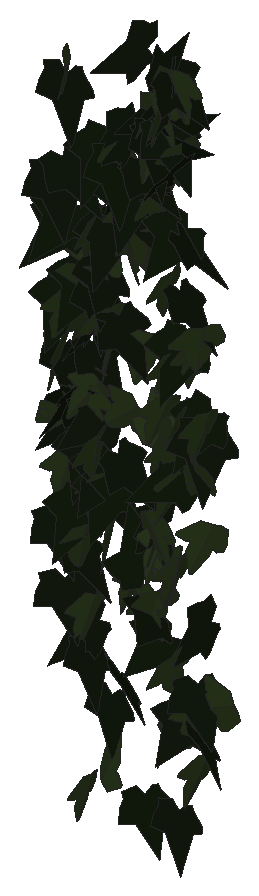
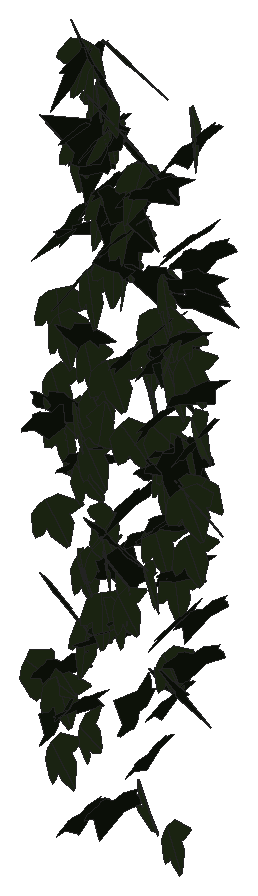
# SketchUp Ruby script. Lengths in inches.
U = 1.inch
M = Sketchup.active_model
def pt(a) = Geom::Point3d.new(a.map { |v| v * U })
def face(e, loops, mat)
  f = e.add_face(loops[0].map { |a| pt(a) })
  loops[1..].each { |l| e.add_face(l.map { |a| pt(a) }).erase! }
  f.material = f.back_material = mat if mat
  f
end
# faces: each face lists its corners as indices into pts; further lists are holes
def faces(e, pts, list, mat = nil) = list.each { |f| face(e, (f[0].is_a?(Array) ? f : [f]).map { |l| l.map { |i| pts[i] } }, mat) }
# xy, xz, yz: faces in a plane at the given z, y or x. An outline is a flat list of corners, or four numbers for a rectangle; further outlines are holes
def ring(l) = l.size == 4 ? [[l[0], l[1]], [l[2], l[1]], [l[2], l[3]], [l[0], l[3]]] : l.each_slice(2).to_a
def flat(e, list, mat, &to3) = list.each { |f| face(e, (f[0].is_a?(Array) ? f : [f]).map { |l| ring(l).map { |u, v| to3.(u, v) } }, mat) }
def xy(e, z, list, mat = nil) = flat(e, list, mat) { |x, y| [x, y, z] }
def xz(e, y, list, mat = nil) = flat(e, list, mat) { |x, z| [x, y, z] }
def yz(e, x, list, mat = nil) = flat(e, list, mat) { |y, z| [x, y, z] }
def lines(e, pts, list) = list.each { |a, b| e.add_line(pt(pts[a]), pt(pts[b])) }
# prism: a flat outline (further loops are holes) pulled along v
def prism(e, loops, v, mat = nil)
  f = face(e, loops, mat); d = Geom::Vector3d.new(v.map { |x| x * U })
  f.pushpull(f.normal.samedirection?(d) ? d.length : -d.length)
end
def box(e, o, s, mat = nil) = prism(e, [[o, [o[0] + s[0], o[1], o[2]], [o[0] + s[0], o[1] + s[1], o[2]], [o[0], o[1] + s[1], o[2]]]], [0, 0, s[2]], mat)
def at(x, y, z, deg = 0) = Geom::Transformation.translation(pt([x, y, z])) * Geom::Transformation.rotation(ORIGIN, Z_AXIS, deg.degrees)
def axes(o, x, y, z) = Geom::Transformation.new([*x, 0, *y, 0, *z, 0, *pt(o).to_a, 1])
def part(name) = M.definitions.add(name)
# library, detail: a bought-in or finely detailed component or shape, given as its bounding box
def library(name, o, s) = part(name).tap { |d| box(d.entities, o, s) }
def detail(e, o, s) = box(e.add_group.entities, o, s)
def put(e, d, t, mat = nil) = e.add_instance(d, t).tap { |i| i.material = mat if mat }
def group(e, t, mat = nil) = e.add_group.tap { |g| g.transformation = t; g.material = mat if mat }.entities
root = M.entities
M.materials.add("efeu1").color = [18, 25, 13]
M.materials.add("efeu2").color = [43, 57, 29]
c1 = part("ivyleaf_10")
p = [[0,0.5,-0.03],[-0.0625,2.02,-0.43],[-0.19,2.01,-0.46],[-0.54,1.05,-0.29],[-0.52,0.625,-0.18],[-0.83,0.76,-0.28],
  [-1.16,0.64,-0.33],[-1.15,0.33,-0.24],[-0.77,-0.39,0.02],[-0.3,-0.51,0.16],[0.04,-0.48,0.23],[-0.02,2.01,-0.4375],
  [-0.06,2.01,-0.43],[0.04,-0.49,0.23],[0.67,-0.49,0.14],[1.38,0.36,-0.2],[1.375,0.51,-0.24],[0.81,0.65,-0.19],
  [0.62,0.59,-0.15],[0.6,1.09,-0.28],[0.5,1.23,-0.31]]
faces(c1.entities,p,[[0,1,2,3,4,5,6,7,8,9,10],[11,12,0,13,14,15,16,17,18,19,20]],"efeu2")
c2 = part("ivyleaf_9")
p = [[1.54,2.16,1.25],[1.36,2.04,1.19],[-0.21,0.99,0.68],[-0.71,1.11,0.82],[-0.85,0.86,0.67],[-0.8,0.17,0.21],
  [-0.9,-0.01,0.1],[-0.67,-0.16,-0.02],[-0.08,-0.08,-0.05],[-0.03,-0.6,-0.4],[0.65,-0.88,-0.66],[0.83,-0.6,-0.49],
  [1.29,-0.42,-0.43],[1.8125,-0.07,-0.26],[1.21,0.44,0.15]]
faces(c2.entities,p,[[0,1,2,3,4,5,6,7,8,9,10,11,12,13,14]],"efeu1")
put(root,c1,axes([526.16,131.21,239.89],[0.45745,-0.87487,-0.09808],[0.01557,0.11855,-0.98488],[0.88021,0.45257,0.06839]))
put(root,c1,axes([522.93,131.16,223.58],[0.0269,-0.92071,-0.14302],[0.00472,0.14321,-0.92106],[0.93174,0.02586,0.00879]))
put(root,c2,axes([521.15,131.58,239.56],[0.07665,-0.98925,-0.02502],[-0.01925,0.0236,-0.99206],[0.98938,0.0771,-0.01737]))
put(root,c2,axes([524.41,131.73,235.49],[-0.2445,-0.93887,0.09298],[-0.00632,-0.09442,-0.97003],[0.94344,-0.24395,0.0176]))
put(root,c1,axes([526.94,131.03,214.93],[-0.1751,-0.89884,-0.3085],[0.08375,0.29787,-0.91543],[0.94661,-0.19262,0.02393]))
put(root,c2,axes([525.29,131.9,216.17],[-0.26022,-0.64301,0.58185],[0.22645,-0.63679,-0.60245],[0.8371,-0.02762,0.34385]))
put(root,c1,axes([526.52,130.88,225.14],[0.21684,-0.73874,-0.54662],[0.13314,0.58096,-0.73233],[0.90929,0.09111,0.23758]))
put(root,c2,axes([523.6875,131.62,236.61],[-0.02137,-0.98061,-0.09477],[0.00149,0.09476,-0.98084],[0.98517,-0.02142,-0.00057]))
put(root,c2,axes([525.63,131.67,238.39],[0.16649,-0.97049,0.06718],[-0.00025,-0.0682,-0.98459],[0.97281,0.16608,-0.01175]))
put(root,c2,axes([522.27,131.58,213.65],[0.14457,-0.87641,-0.02007],[-0.00231,0.01996,-0.88825],[0.87664,0.14458,0.00097]))
put(root,c2,axes([523.02,131.86,236.97],[-0.50649,-0.83413,0.08884],[0.03508,-0.12475,-0.97129],[0.83811,-0.49886,0.09434]))
put(root,c2,axes([521.68,131.92,219.92],[-0.42513,-0.8034,0.19731],[-0.05961,-0.19151,-0.90823],[0.82512,-0.42778,0.03605]))
put(root,c2,axes([526.93,130.72,237.33],[0.00765,0.95187,0.24437],[-0.01575,0.24446,-0.95175],[-0.98261,0.00349,0.01716]))
put(root,c2,axes([525.27,131.4,242.33],[-0.87542,0.45236,0.16553],[-0.20762,-0.04451,-0.97638],[-0.43466,-0.88982,0.133]))
put(root,c1,axes([521.4,131.19,240.36],[0.5028,-0.78984,-0.35606],[-0.0926,0.36033,-0.93007],[0.86143,0.49975,0.10784]))
put(root,c2,axes([524.31,131.49,238.12],[-0.94168,0.27966,-0.00731],[0.0064,-0.00414,-0.98232],[-0.27968,-0.9417,0.00214]))
put(root,c1,axes([528.17,131.58,226.2],[-0.00795,-0.92129,0.17894],[0.0119,-0.17903,-0.92123],[0.93844,-0.00554,0.01319]))
put(root,c2,axes([525.91,132.05,215.29],[-0.59192,-0.5599,0.38395],[-0.0699,-0.45642,-0.77335],[0.67529,-0.53802,0.25649]))
put(root,c1,axes([522.13,131.42,219.07],[-0.22865,-0.88154,-0.0035],[0.00118,0.00331,-0.91071],[0.88154,-0.22865,0.00032]))
put(root,c2,axes([526.93,132.04,223.02],[-0.63851,-0.36043,0.60223],[-0.40913,-0.47038,-0.71529],[0.57026,-0.74103,0.16112]))
put(root,c1,axes([526.91,131.29,241.55],[-0.98612,0.08208,-0.12222],[0.1162,-0.07435,-0.98746],[-0.0904,-0.99088,0.06397]))
put(root,c2,axes([521.21,131.92,233.41],[-0.77924,-0.54246,0.1085],[-0.077,-0.07924,-0.94923],[0.54782,-0.78275,0.0209]))
put(root,c1,axes([525.39,131.63,238.45],[0.05897,0.89388,-0.41727],[-0.03025,-0.41618,-0.89582],[-0.98601,0.06622,0.00253]))
put(root,c2,axes([522.79,132.1,224.45],[-0.54463,-0.55878,0.4979],[-0.30959,-0.39242,-0.77905],[0.68139,-0.62492,0.044]))
put(root,c1,axes([522.49,131.91,225.86],[-0.28668,-0.62588,0.62813],[-0.19889,-0.59793,-0.68657],[0.86413,-0.34526,0.05036]))
put(root,c1,axes([526.04,131.75,226.17],[-0.13417,-0.8722,0.31137],[-0.05156,-0.3071,-0.88245],[0.92468,-0.14368,-0.00403]))
put(root,c1,axes([526.51,131.91,222.6875],[0.07964,-0.78186,0.49958],[0.05181,-0.49688,-0.78591],[0.92639,0.095,0.00101]))
put(root,c1,axes([521.16,131.79,229.31],[-0.12945,-0.90458,0.32863],[0.0044,-0.33215,-0.91251],[0.96241,-0.12015,0.04838]))
put(root,c1,axes([523.3,131.48,229.36],[-0.30349,-0.88514,-0.09861],[0.03706,0.09153,-0.93571],[0.88984,-0.3057,0.00534]))
put(root,c2,axes([526.84,132.17,211.86],[-0.40832,-0.71301,0.34579],[-0.03265,-0.37353,-0.80876],[0.79176,-0.38311,0.14497]))
put(root,c2,axes([520.53,131.76,234.875],[-0.15825,-0.9116,-0.31859],[0.08073,0.30922,-0.92489],[0.96229,-0.17585,0.0252]))
put(root,c2,axes([522.81,131.59,229.21],[-0.72667,0.60822,-0.28042],[0.18796,-0.21195,-0.94677],[-0.64284,-0.74951,0.04017]))
put(root,c1,axes([528.01,131.35,224.09],[-0.82191,0.08539,0.49093],[-0.48818,0.05186,-0.82633],[-0.0999,-0.95595,-0.00098]))
put(root,c2,axes([520.98,131.98,232.76],[-0.89275,-0.32041,0.09017],[-0.06278,-0.09139,-0.94631],[0.32688,-0.89263,0.06452]))
put(root,c1,axes([525.48,131.58,220.68],[-0.74831,0.31004,-0.44507],[0.37399,-0.25436,-0.80599],[-0.39287,-0.83268,0.08049]))
put(root,c2,axes([525.11,131.65,207.88],[0.00386,-0.78759,-0.37309],[-0.02363,0.37286,-0.78735],[0.87117,0.0136,-0.0197]))
put(root,c2,axes([523.03,132.11,221.29],[-0.38986,-0.8427,0.09054],[-0.00558,-0.09711,-0.92783],[0.84753,-0.38828,0.03554]))
put(root,c2,axes([523.59,131.98,212.78],[0.41557,-0.67224,0.50939],[0.29811,-0.41414,-0.78975],[0.789,0.51055,0.03009]))
put(root,c2,axes([521.77,132.22,230.41],[-0.51524,-0.78089,0.17721],[-0.02749,-0.19336,-0.93195],[0.80027,-0.5094,0.08209]))
put(root,c2,axes([521.85,131.46,225.18],[0.47545,0.57943,-0.60516],[-0.3701,-0.47899,-0.7494],[-0.75165,0.60236,-0.01379]))
put(root,c1,axes([522.04,131.8,207.45],[0.13598,-0.85125,0.13331],[0.04162,-0.12832,-0.8618],[0.86062,0.14071,0.02061]))
put(root,c1,axes([524.52,131.97,218.43],[0.015,-0.36595,-0.87914],[0.7619,-0.52283,0.23064],[-0.57124,-0.70694,0.28452]))
put(root,c1,axes([522.04,132,215.5],[-0.09112,-0.80566,0.38234],[0.12785,-0.39217,-0.79589],[0.88257,-0.02637,0.15477]))
put(root,c2,axes([520.88,131.81,216.23],[-0.11344,-0.81154,-0.36458],[0.13083,0.34832,-0.81605],[0.88,-0.1564,0.07433]))
put(root,c1,axes([522.06,131.59,225.28],[-0.88673,-0.05479,-0.25274],[0.25696,-0.08491,-0.88314],[0.02915,-0.91813,0.09676]))
put(root,c2,axes([526,131.62,239.68],[-0.8352,0.49732,0.17445],[-0.17095,0.05358,-0.9712],[-0.49853,-0.85154,0.04077]))
put(root,c1,axes([525.6,131.62,239.86],[-0.88626,0.22484,-0.37665],[0.3452,-0.16642,-0.9116],[-0.27066,-0.94848,0.07067]))
put(root,c2,axes([526.73,131.37,241.62],[0.35927,-0.60975,-0.70099],[-0.28636,0.64231,-0.70547],[0.88384,0.45596,0.05637]))
put(root,c2,axes([526.57,132.33,234.09],[-0.66559,-0.65359,0.21848],[0.02765,-0.32882,-0.89947],[0.68859,-0.61857,0.2473]))
put(root,c2,axes([528.21,131.83,216.87],[-0.94,0.24426,-0.14113],[0.13769,-0.03125,-0.9712],[-0.24621,-0.95002,-0.00434]))
put(root,c1,axes([527.9375,131.73,230],[-0.45804,-0.84692,0.04673],[-0.00526,-0.05027,-0.96265],[0.84819,-0.45767,0.01927]))
put(root,c2,axes([526.875,132.06,229.15],[-0.76516,-0.54241,-0.20354],[0.15941,0.12705,-0.93784],[0.55697,-0.78151,-0.0112]))
put(root,c2,axes([525.85,131.5625,240.76],[-0.39631,0.65191,0.63481],[0.32548,-0.54503,0.76291],[0.84972,0.51282,0.00384]))
put(root,c2,axes([522.47,132.37,221.61],[-0.3476,-0.74237,0.40176],[0.02115,-0.44201,-0.79845],[0.84384,-0.29472,0.18551]))
put(root,c1,axes([521.88,131.68,230.72],[-0.82619,-0.45765,0.09285],[-0.07662,-0.05327,-0.94443],[0.46064,-0.82969,0.00943]))
put(root,c1,axes([523.2,131.77,227.91],[0.55829,-0.75308,-0.07967],[-0.01961,0.08458,-0.93681],[0.75703,0.55756,0.03449]))
put(root,c1,axes([520.51,132.02,226.89],[0.47606,-0.79399,0.25862],[0.11349,-0.23342,-0.92551],[0.8273,0.48891,-0.02186]))
put(root,c2,axes([523.74,131.76,229.28],[0.24314,-0.84332,-0.39837],[-0.01942,0.40702,-0.87347],[0.93247,0.22837,0.08568]))
put(root,c2,axes([521.61,132.02,225.21],[-0.4288,0.51904,-0.66568],[0.19953,-0.66316,-0.64561],[-0.82019,-0.43268,0.19096]))
put(root,c2,axes([525.13,131.61,218.29],[-0.86408,-0.35779,0.20506],[0.22083,0.00062,0.93163],[-0.34828,0.88808,0.08196]))
put(root,c1,axes([526.21,131.9,228.19],[0.03039,-0.94512,0.06097],[0.01164,-0.06063,-0.94556],[0.94701,0.03108,0.00967]))
put(root,c2,axes([526.07,131.85,238.75],[0.10466,-0.87795,-0.42366],[0.03759,0.42941,-0.88058],[0.9741,0.07776,0.0795]))
put(root,c1,axes([525.375,132.37,219.46],[-0.20063,-0.60862,0.64247],[0.30758,-0.66565,-0.53453],[0.8298,0.09959,0.35347]))
put(root,c2,axes([523.08,132.16,233.2],[-0.74501,-0.52187,-0.30455],[0.24682,0.17847,-0.9096],[0.55153,-0.78482,-0.00433]))
put(root,c2,axes([525.44,131.79,237.79],[0.39932,-0.14629,0.88705],[0.83328,-0.30414,-0.42527],[0.3375,0.92402,0.00046]))
put(root,c2,axes([520.83,131.81,235.52],[0.41234,-0.81669,-0.35429],[0.08045,0.42304,-0.88153],[0.88659,0.34144,0.24476]))
put(root,c1,axes([526.29,131.68,240.87],[-0.51079,0.83488,0.13187],[-0.2874,-0.02666,-0.94446],[-0.79486,-0.52686,0.25675]))
put(root,c1,axes([523.78,131.625,237.16],[-0.33393,-0.85286,-0.36926],[0.19404,0.31975,-0.91397],[0.90889,-0.38161,0.05945]))
put(root,c1,axes([524.67,131.32,232.79],[-0.43643,0.5177,0.7093],[-0.50629,0.49883,-0.6756],[-0.71749,-0.6669,0.04528]))
put(root,c2,axes([524.81,131.6875,236.86],[0.46032,-0.70377,-0.5022],[-0.09143,0.52613,-0.82111],[0.85973,0.43277,0.18157]))
put(root,c2,axes([522.29,132.07,214.79],[-0.99073,0.12903,-0.01038],[0.00973,-0.0057,-0.99908],[-0.12908,-0.99077,0.00439]))
put(root,c2,axes([527.52,131.99,213.62],[-0.09335,-0.79826,-0.4047],[0.06053,0.40033,-0.80361],[0.89293,-0.11059,0.01216]))
put(root,c1,axes([524.22,131.93,225.2],[-0.57256,-0.14106,0.73762],[-0.70706,-0.2113,-0.58925],[0.25306,-0.90953,0.02249]))
put(root,c2,axes([524.66,131.9,236.22],[-0.55008,0.75007,-0.30003],[0.00637,-0.35894,-0.90903],[-0.80783,-0.51358,0.19713]))
put(root,c2,axes([522.39,132.43,230.75],[-0.05316,-0.92287,0.20804],[0.1046,-0.21282,-0.91736],[0.94022,-0.0285,0.11382]))
put(root,c1,axes([521.75,132.09,228.8],[0.21998,-0.91822,0.11871],[0.01005,-0.11964,-0.94404],[0.92581,0.21948,-0.01796]))
put(root,c2,axes([521.72,132.41,222.66],[-0.31993,-0.86118,0.0712],[-0.01817,-0.0692,-0.91867],[0.86393,-0.32037,0.00704]))
put(root,c1,axes([527.4375,132.06,229.16],[-0.05587,-0.94317,0.10208],[0.02103,-0.10346,-0.94444],[0.94844,-0.05326,0.02696]))
put(root,c2,axes([527.74,132.29,225.14],[-0.28712,-0.94966,-0.20046],[0.07392,0.18705,-0.99198],[0.96777,-0.29604,0.0163]))
put(root,c2,axes([522.18,132.35,229.75],[0.06543,-0.93776,0.07241],[0.00803,-0.07203,-0.94004],[0.94052,0.06586,0.00299]))
put(root,c1,axes([522.54,132.1,221.26],[-0.15307,-0.90496,0.15875],[-0.02192,-0.15729,-0.9178],[0.91851,-0.15456,0.00456]))
put(root,c1,axes([522.86,132.2,219.22],[0.50438,-0.72281,0.29148],[0.19903,-0.21623,-0.8806],[0.75353,0.54093,0.03748]))
put(root,c1,axes([525.9,132.19,223.96],[0.03963,-0.89494,0.25146],[-0.02115,-0.2525,-0.89527],[0.92935,0.03242,-0.0311]))
put(root,c2,axes([527.35,132.34,211.3],[0.4252,-0.75365,0.41974],[0.20005,-0.36905,-0.8653],[0.83914,0.46987,-0.00639]))
put(root,c2,axes([520.39,132.31,226.48],[0.21578,-0.9131,0.06439],[0.00758,-0.06437,-0.93822],[0.91534,0.21579,-0.00741]))
put(root,c1,axes([524.71,132.02,216.78],[-0.6964,0.29604,-0.53495],[0.44949,-0.30174,-0.75213],[-0.41445,-0.82468,0.08316]))
put(root,c2,axes([526.74,131.95,231.37],[0.54071,-0.75368,-0.2417],[-0.05278,0.25773,-0.92174],[0.78972,0.53326,0.10388]))
put(root,c2,axes([526.91,131.73,234.12],[0.75203,-0.51566,-0.29418],[-0.11471,0.33961,-0.88854],[0.58248,0.73264,0.20482]))
put(root,c1,axes([527.52,132.125,212.52],[-0.37131,-0.78897,0.20128],[-0.04473,-0.20112,-0.87086],[0.81301,-0.3714,0.04401]))
put(root,c1,axes([524.07,132.32,217.63],[0.01296,-0.80066,0.39776],[0.13131,-0.39178,-0.79291],[0.88432,0.06991,0.11191]))
put(root,c1,axes([525.39,131.91,219.77],[0.45068,-0.75495,-0.23389],[-0.07471,0.22735,-0.87778],[0.78681,0.45402,0.05063]))
put(root,c1,axes([524.14,132.0625,234.55],[-0.19908,-0.94887,0.03635],[0.00608,-0.03841,-0.96944],[0.94955,-0.19869,0.01383]))
put(root,c1,axes([526.23,132.24,218.65],[0.03134,-0.89479,0.23589],[0.05631,-0.23374,-0.89413],[0.92365,0.04461,0.0465]))
put(root,c1,axes([527.85,132.3,220.65],[-0.46739,-0.68114,0.40284],[-0.09467,-0.41637,-0.81385],[0.78566,-0.45538,0.14158]))
put(root,c1,axes([525.45,131.97,217.01],[-0.38793,-0.82469,-0.05564],[0.0131,0.05532,-0.91131],[0.82647,-0.38798,-0.01167]))
put(root,c2,axes([526.23,132.36,207.24],[0.04152,-0.88048,0.00723],[-0.00034,-0.00725,-0.88146],[0.88051,0.04152,-0.00068]))
put(root,c1,axes([525.85,132.51,211.24],[0.21175,-0.65276,0.62987],[0.29411,-0.56245,-0.68177],[0.8581,0.35386,0.07825]))
put(root,c1,axes([525.67,131.88,224.57],[0.85928,0.41996,0.12321],[-0.1129,-0.04959,0.9564],[0.42285,-0.86665,0.00498]))
put(root,c1,axes([526.59,131.96,237.88],[-0.2684,-0.92636,-0.14907],[0.01537,0.15069,-0.96408],[0.93815,-0.2675,-0.02686]))
put(root,c2,axes([522.72,132.46,211.26],[0.08802,-0.88571,0.109],[-0.00559,-0.11007,-0.88992],[0.89237,0.08667,-0.01633]))
put(root,c2,axes([520.11,132.19,218.7],[0.10349,-0.84045,-0.29216],[0.02606,0.29686,-0.84476],[0.88941,0.08909,0.05875]))
put(root,c1,axes([520.49,131.93,224.07],[-0.7707,-0.34323,-0.36147],[0.36816,0.05674,-0.83886],[0.33604,-0.84937,0.09003]))
put(root,c2,axes([521.24,132.18,223.99],[-0.8607,0.30878,-0.06585],[0.05091,-0.05298,-0.91383],[-0.31159,-0.86159,0.0326]))
put(root,c2,axes([527.71,132.45,225.92],[-0.8602,-0.36913,-0.1268],[0.12018,0.04145,-0.93601],[0.37134,-0.8685,0.00922]))
put(root,c1,axes([525.93,132.13,231.7],[0.07253,-0.94381,-0.07882],[0.00398,0.07935,-0.94654],[0.94709,0.07194,0.01002]))
put(root,c1,axes([522.06,132.14,232.89],[0.20649,-0.94188,-0.09465],[0.01799,0.10076,-0.96346],[0.94646,0.20357,0.03897]))
put(root,c1,axes([522.75,132.16,207.98],[0.72709,-0.50813,-0.25575],[0.21536,-0.13827,0.88699],[-0.52652,-0.75825,0.00964]))
put(root,c2,axes([520.37,132.71,228.86],[-0.42112,-0.82982,0.15585],[0.03517,-0.19125,-0.92327],[0.8436,-0.40627,0.11629]))
put(root,c1,axes([528.7,132.26,213.05],[-0.31911,-0.0873,0.93419],[-0.87123,-0.33871,-0.32926],[0.34829,-0.92727,0.03232]))
put(root,c2,axes([524.14,132.11,234.55],[0.41222,-0.80483,-0.35202],[-0.00287,0.38761,-0.88958],[0.87844,0.37895,0.16228]))
put(root,c2,axes([521.28,132.13,217.95],[0.42394,-0.76707,-0.2839],[-0.01146,0.31417,-0.86596],[0.81785,0.40202,0.13503]))
put(root,c2,axes([523.76,131.97,233.89],[0.71877,0.62064,-0.17745],[0.1413,0.10786,0.94959],[0.62985,-0.73245,-0.01053]))
put(root,c1,axes([525.47,131.98,235.58],[-0.07732,-0.91247,-0.32673],[0.10281,0.3182,-0.91297],[0.96373,-0.10715,0.07118]))
put(root,c2,axes([523.5625,131.97,222.8],[0.41384,-0.65445,-0.53289],[-0.14516,0.52947,-0.76298],[0.83139,0.41822,0.13204]))
put(root,c1,axes([527.31,132.51,209.79],[0.06566,-0.88374,0.32845],[0.0209,-0.3278,-0.88617],[0.94257,0.06883,-0.00323]))
put(root,c1,axes([520.6,132.44,221.52],[-0.25815,-0.83034,0.27287],[0.02529,-0.2915,-0.86311],[0.87366,-0.23691,0.10561]))
put(root,c1,axes([522.18,132.35,231.42],[-0.83773,-0.33257,0.30291],[-0.18675,-0.32539,-0.87372],[0.40925,-0.82925,0.22136]))
put(root,c2,axes([525.49,131.81,238.0625],[0.07887,0.02213,0.98086],[0.97647,0.09385,-0.08063],[-0.09534,0.97954,-0.01443]))
put(root,c1,axes([521.9,132.13,230.14],[-0.57217,0.73013,-0.19511],[0.14684,-0.13265,-0.92702],[-0.74134,-0.58979,-0.03304]))
put(root,c1,axes([526.48,132.24,225.63],[0.3274,-0.87046,-0.11063],[-0.02675,0.10813,-0.92991],[0.87706,0.32824,0.01293]))
put(root,c1,axes([520.76,132.39,223.64],[-0.58228,-0.63775,0.3283],[-0.19503,-0.26616,-0.86295],[0.69027,-0.61318,0.03312]))
put(root,c2,axes([522,132.25,227.25],[0.35018,-0.8096,-0.30899],[0.00819,0.33635,-0.87198],[0.86652,0.324,0.13312]))
put(root,c2,axes([525.42,132.05,220.24],[-0.56539,0.45589,0.56706],[-0.51963,0.24966,-0.71882],[-0.50929,-0.76084,0.1039]))
put(root,c1,axes([524.72,132.16,233.25],[-0.32765,-0.8956,-0.12697],[0.01476,0.12974,-0.95316],[0.90443,-0.32657,-0.03045]))
put(root,c1,axes([524.65,132.47,228.2],[-0.58595,-0.66588,0.30897],[-0.07902,-0.33582,-0.8736],[0.72981,-0.57098,0.15347]))
put(root,c1,axes([526.03,132.53,218.76],[0.61267,-0.58752,0.35337],[0.2543,-0.24537,-0.84885],[0.6367,0.66335,-0.00101]))
